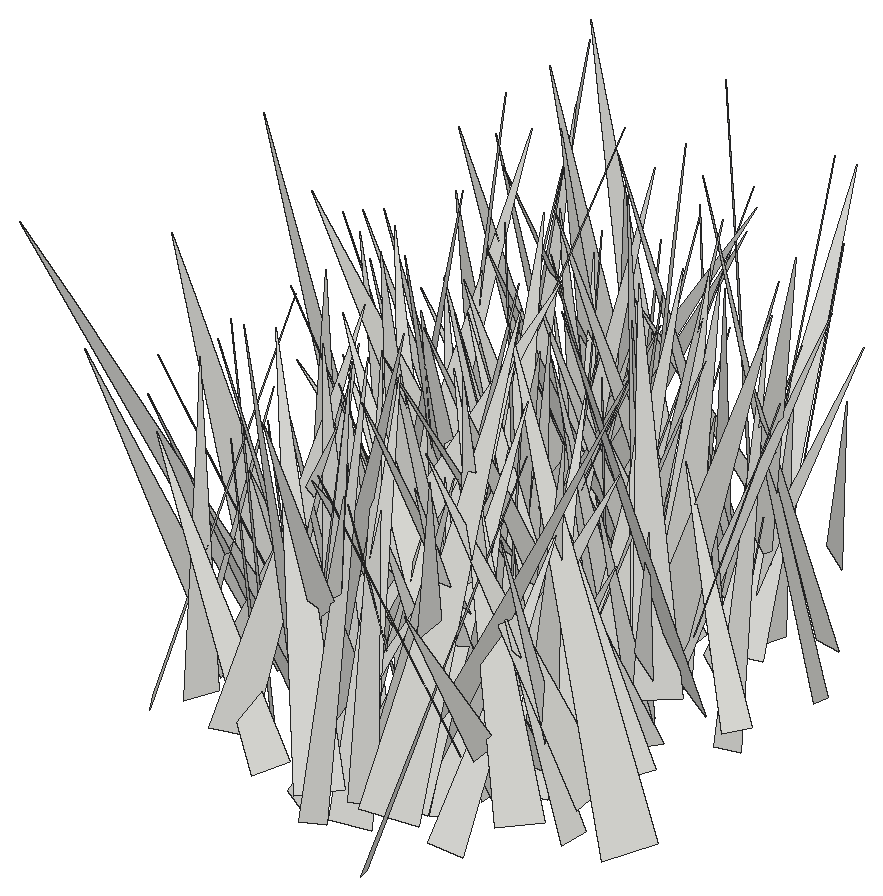
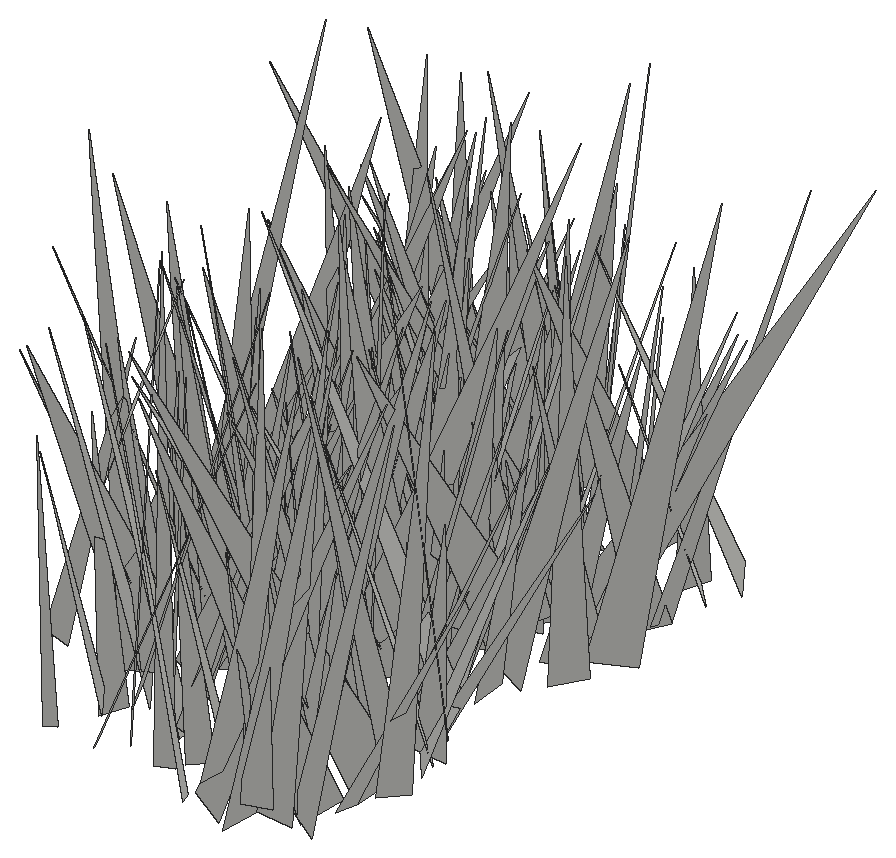
# SketchUp Ruby script. Lengths in inches.
U = 1.inch
M = Sketchup.active_model
def pt(a) = Geom::Point3d.new(a.map { |v| v * U })
def face(e, loops, mat)
  f = e.add_face(loops[0].map { |a| pt(a) })
  loops[1..].each { |l| e.add_face(l.map { |a| pt(a) }).erase! }
  f.material = f.back_material = mat if mat
  f
end
# faces: each face lists its corners as indices into pts; further lists are holes
def faces(e, pts, list, mat = nil) = list.each { |f| face(e, (f[0].is_a?(Array) ? f : [f]).map { |l| l.map { |i| pts[i] } }, mat) }
# xy, xz, yz: faces in a plane at the given z, y or x. An outline is a flat list of corners, or four numbers for a rectangle; further outlines are holes
def ring(l) = l.size == 4 ? [[l[0], l[1]], [l[2], l[1]], [l[2], l[3]], [l[0], l[3]]] : l.each_slice(2).to_a
def flat(e, list, mat, &to3) = list.each { |f| face(e, (f[0].is_a?(Array) ? f : [f]).map { |l| ring(l).map { |u, v| to3.(u, v) } }, mat) }
def xy(e, z, list, mat = nil) = flat(e, list, mat) { |x, y| [x, y, z] }
def xz(e, y, list, mat = nil) = flat(e, list, mat) { |x, z| [x, y, z] }
def yz(e, x, list, mat = nil) = flat(e, list, mat) { |y, z| [x, y, z] }
def lines(e, pts, list) = list.each { |a, b| e.add_line(pt(pts[a]), pt(pts[b])) }
# prism: a flat outline (further loops are holes) pulled along v
def prism(e, loops, v, mat = nil)
  f = face(e, loops, mat); d = Geom::Vector3d.new(v.map { |x| x * U })
  f.pushpull(f.normal.samedirection?(d) ? d.length : -d.length)
end
def box(e, o, s, mat = nil) = prism(e, [[o, [o[0] + s[0], o[1], o[2]], [o[0] + s[0], o[1] + s[1], o[2]], [o[0], o[1] + s[1], o[2]]]], [0, 0, s[2]], mat)
def at(x, y, z, deg = 0) = Geom::Transformation.translation(pt([x, y, z])) * Geom::Transformation.rotation(ORIGIN, Z_AXIS, deg.degrees)
def axes(o, x, y, z) = Geom::Transformation.new([*x, 0, *y, 0, *z, 0, *pt(o).to_a, 1])
def part(name) = M.definitions.add(name)
# library, detail: a bought-in or finely detailed component or shape, given as its bounding box
def library(name, o, s) = part(name).tap { |d| box(d.entities, o, s) }
def detail(e, o, s) = box(e.add_group.entities, o, s)
def put(e, d, t, mat = nil) = e.add_instance(d, t).tap { |i| i.material = mat if mat }
def group(e, t, mat = nil) = e.add_group.tap { |g| g.transformation = t; g.material = mat if mat }.entities
root = M.entities
c1 = part("fur_instance\#9")
p = [[0.8125,0,1.79],[0.67,-0.02,1.48],[0,-0.11,0],[0,0.11,0]]
faces(c1.entities,p,[[0,1,2,3]])
put(root,c1,axes([67.05,77.16,-27.1],[-1.39061,-8.04384,0.83594],[-7.45661,0.94696,-3.29214],[-3.13068,1.31752,7.46987]))
put(root,c1,axes([64.83,79.17,-27.1],[4.91943,-4.73173,2.30235],[-4.40019,-5.42749,-1.75256],[-2.8859,0.2095,6.59686]))
put(root,c1,axes([66.79,85.26,-28.22],[-4.61833,-3.74237,0.73758],[-3.79853,4.40694,-1.4242],[-0.34716,1.56584,5.77113]))
put(root,c1,axes([65.1875,76.49,-27.1],[-6.16239,-2.08969,1.53365],[-1.42213,6.03269,2.50561],[2.16712,-1.98337,6.00531]))
put(root,c1,axes([66.03,78.65,-27.1],[-3.26059,-4.43586,0.10579],[-4.43536,3.26207,0.0775],[0.12511,0.03932,5.50476]))
put(root,c1,axes([66.9375,81.38,-27.1],[-2.69995,-7.06667,2.40673],[-7.39529,2.18224,-1.88876],[-1.01973,2.88442,7.32531]))
put(root,c1,axes([66.75,88.64,-28.22],[-4.32306,0.06447,0.02072],[0.06687,4.27292,0.65655],[0.01068,-0.65679,4.2734]))
put(root,c1,axes([66.48,82.625,-27.1],[-5.31115,0.249,1.00047],[0.14264,5.37711,-0.58108],[1.02108,0.54405,5.28514]))
put(root,c1,axes([67.13,84.4,-28.22],[-4.70731,-0.314,0.0439],[-0.28456,4.4722,1.47573],[0.13983,-1.46975,4.48103]))
put(root,c1,axes([67.86,85.51,-28.22],[-6.00367,-1.40851,0.07652],[-1.40991,5.98159,-0.51624],[-0.04369,0.52005,6.14503]))
put(root,c1,axes([67.36,77.11,-28.22],[-2.53227,-4.93937,0.36335],[-4.86121,2.40071,-1.24381],[-0.94765,0.88376,5.4095]))
put(root,c1,axes([65.32,74.46,-27.1],[3.04107,3.48011,0.59696],[3.3547,-3.09349,0.94446],[-1.10161,0.1866,4.52408]))
put(root,c1,axes([65.85,74.29,-27.1],[-4.75498,1.70819,1.94206],[1.76287,5.11453,-0.18234],[1.89256,-0.47231,5.04921]))
put(root,c1,axes([66.79,84.88,-28.22],[-0.91318,4.58049,0.90258],[4.61205,0.74242,0.89849],[-0.72428,-1.04754,4.5834]))
put(root,c1,axes([65,73.07,-27.1],[5.18703,3.91751,0.7095],[3.72248,-5.18551,1.41748],[-1.41191,0.72053,6.34373]))
put(root,c1,axes([64.89,88.83,-27.1],[6.40589,-1.32849,1.4611],[-0.83624,-6.31798,-2.07823],[-1.78897,-1.80373,6.20333]))
put(root,c1,axes([65.13,80.71,-27.1],[5.79339,-2.08626,1.56673],[-1.97661,-6.00002,-0.68061],[-1.70297,-0.13319,6.11985]))
put(root,c1,axes([67.12,90.14,-28.22],[-3.32824,-5.52708,1.61735],[-5.74671,3.30884,-0.51825],[0.37393,1.65668,6.43096]))
put(root,c1,axes([67.9,75.06,-28.22],[-4.69579,-3.74143,2.09942],[-4.25802,4.44495,-1.60248],[0.52452,2.58851,5.78625]))
put(root,c1,axes([66.11,78.47,-27.1],[0.58745,4.61701,1.14714],[4.75417,-0.52722,-0.31264],[0.17496,-1.17604,4.64372]))
put(root,c1,axes([66.54,86.9,-27.1],[6.51752,3.06728,2.32468],[2.5593,-6.86862,1.88745],[-2.87443,0.8392,6.95153]))
put(root,c1,axes([68.79,73.77,-28.22],[-4.48303,2.72425,0.35571],[2.72908,4.33728,1.17718],[-0.3165,-1.18832,5.11208]))
put(root,c1,axes([66.82,75.65,-27.1],[-2.76326,-3.0585,1.38467],[-3.15346,2.97986,0.28892],[1.15213,0.82059,4.11176]))
put(root,c1,axes([68.75,81.83,-28.22],[-3.88022,2.75048,0.41463],[2.75578,3.70465,1.21426],[-0.37781,-1.22622,4.59857]))
put(root,c1,axes([67.08,84.48,-28.22],[4.3588,4.87451,1.02077],[4.50794,-4.43827,1.9448],[-2.11691,0.58556,6.24322]))
put(root,c1,axes([68.4375,84.53,-28.22],[-6.28754,-2.52373,1.27093],[-2.51372,6.41179,0.29625],[1.29062,0.19325,6.76865]))
put(root,c1,axes([66.24,84.8125,-27.1],[5.70767,4.90783,2.44546],[5.23724,-5.92496,-0.33273],[-1.62433,-1.85811,7.52021]))
put(root,c1,axes([67.25,78.6,-28.22],[3.46395,-3.11936,0.86631],[-2.7787,-3.51575,-1.54862],[-1.66124,-0.62369,4.39672]))
put(root,c1,axes([68.02,78.52,-27.1],[-3.33951,2.40161,0.05247],[2.31618,3.24301,-1.02031],[0.63702,0.79874,3.98485]))
put(root,c1,axes([67.73,85.81,-28.22],[1.84085,7.01016,1.12106],[6.97031,-2.00445,1.08846],[-1.34679,-0.79226,7.16563]))
put(root,c1,axes([67.9,82.61,-28.22],[-4.76858,-5.56642,0.65425],[-5.40433,4.79429,1.40014],[1.48534,-0.42682,7.19472]))
put(root,c1,axes([65.24,76.84,-27.1],[2.87453,-4.20489,0.68169],[-4.14129,-2.56592,1.63539],[0.99777,1.46412,4.82385]))
put(root,c1,axes([68.03,79.56,-27.1],[-6.65412,4.03174,0.74119],[3.28122,6.08544,-3.64454],[2.45722,2.79179,6.87384]))
put(root,c1,axes([68.76,87.92,-27.1],[-0.74223,-7.02206,1.66779],[-7.14663,0.48084,-1.156],[-1.00829,1.76103,6.96591]))
put(root,c1,axes([68.6,91.08,-28.22],[6.73753,-0.02978,4.19134],[0.53715,-7.86314,-0.91932],[-4.15689,-1.06433,6.67458]))
put(root,c1,axes([69.54,90.71,-27.1],[-7.31689,1.04904,1.18508],[0.99417,7.40794,-0.41938],[1.23147,0.25252,7.3798]))
put(root,c1,axes([69.73,75.91,-28.22],[-5.59539,-3.44886,0.89561],[-3.54081,5.56848,-0.67808],[0.39927,1.05,6.53783]))
put(root,c1,axes([68.99,87.99,-28.22],[0.68239,3.8164,1.4602],[3.78451,-1.14857,1.23331],[-1.54098,-1.13076,3.67553]))
put(root,c1,axes([69.8,91.05,-28.22],[-3.16334,-6.14078,0.476],[-6.132,3.08971,-0.89149],[-0.57823,0.82883,6.8499]))
put(root,c1,axes([68.99,77.39,-27.1],[-4.42725,-2.60663,1.07476],[-2.66002,4.52485,0.01676],[0.93485,0.53053,5.13759]))
put(root,c1,axes([67.67,79.5,-27.1],[3.15596,1.30372,1.61225],[1.82364,-3.14251,-1.02861],[-0.98659,-1.6383,3.25603]))
put(root,c1,axes([68.04,90.39,-28.22],[-0.95753,-7.17721,1.84222],[-7.39469,1.0444,0.22542],[0.47406,1.79439,7.23729]))
put(root,c1,axes([67.81,73.16,-27.1],[-5.19171,3.73852,1.55221],[3.028,5.26206,-2.54592],[2.68647,1.29382,5.8693]))
put(root,c1,axes([67.7,76.61,-27.1],[-3.39488,-3.98848,1.56761],[-3.7052,3.73666,1.48306],[2.15333,0.14147,5.02331]))
put(root,c1,axes([69.28,82.42,-28.22],[-2.05359,-3.75931,0.63579],[-3.81243,2.01617,-0.39286],[-0.04503,0.74602,4.26559]))
put(root,c1,axes([68.51,90.42,-27.1],[-3.5127,-1.06556,1.8883],[-1.54789,3.74984,-0.76344],[1.51826,1.35772,3.59049]))
put(root,c1,axes([70.71,78.52,-27.1],[-2.20757,6.36235,0.08993],[6.1827,2.12231,1.62203],[-1.50393,-0.61421,6.5362]))
put(root,c1,axes([69.17,87.8,-27.1],[-0.51846,-5.08764,2.15235],[-5.51728,0.36879,-0.45728],[-0.27624,2.18298,5.0935]))
put(root,c1,axes([69.26,77.63,-28.22],[1.73924,-4.25815,2.51532],[-4.74882,-2.1825,-0.41111],[-1.38108,2.14207,4.58125]))
put(root,c1,axes([69.03,76.91,-28.22],[-4.56803,3.68378,2.77525],[4.20348,4.93276,0.37129],[1.89817,-2.05836,5.85656]))
put(root,c1,axes([70.29,86.01,-28.22],[-4.8792,2.06982,0.10093],[1.96371,4.70056,-1.46614],[0.66196,1.31208,5.09325]))
put(root,c1,axes([71,82.37,-27.1],[-7.92224,1.63819,2.17065],[2.33717,7.51957,2.85498],[1.39032,-3.306,7.56932]))
put(root,c1,axes([66.44,84.1,-27.1],[7.55875,3.30018,0.58934],[3.3113,-7.57673,-0.04195],[-0.52327,-0.27436,8.24768]))
put(root,c1,axes([67.67,88.88,-28.22],[1.53162,3.70831,1.75315],[4.01532,-0.97314,-1.44953],[0.83802,-2.1148,3.74116]))
put(root,c1,axes([67.52,91.69,-27.1],[-1.15928,-6.64992,1.1524],[-6.36185,1.46707,2.06591],[2.25307,0.72087,6.42631]))
put(root,c1,axes([69.5625,88.5,-27.1],[-1.29873,-6.18935,0.13887],[-6.18983,1.30082,0.08883],[0.11547,0.11765,6.32352]))
put(root,c1,axes([68.91,87.21,-28.22],[-4.37143,-2.8181,2.86453],[-3.24687,4.97094,-0.06453],[2.3675,1.61389,5.20067]))
put(root,c1,axes([70.03,79.97,-27.1],[-3.79874,-3.55526,0.6962],[-3.51199,3.8615,0.55657],[0.88909,0.06302,5.17306]))
put(root,c1,axes([69.2,74.84,-27.1],[6.14406,2.36607,3.59044],[3.36505,-6.54408,-1.44586],[-2.67694,-2.79567,6.42319]))
put(root,c1,axes([69.2,81.94,-28.22],[2.92591,-1.89098,1.19539],[-1.88086,-3.14489,-0.37117],[-1.21125,0.31559,3.46396]))
put(root,c1,axes([68.77,78.125,-28.22],[7.33246,2.99097,2.42144],[2.72494,-7.71469,1.27771],[-2.71735,0.33456,7.81527]))
put(root,c1,axes([68.36,85.03,-28.22],[3.46775,1.51161,0.84573],[1.722,-3.21287,-1.3182],[-0.18693,-1.55498,3.54578]))
put(root,c1,axes([70.68,85.07,-27.1],[-5.0365,1.95588,2.0654],[2.56555,4.93734,1.5806],[1.22852,-2.29236,5.16658]))
put(root,c1,axes([69.53,80.25,-27.1],[4.70734,-3.12135,0.14145],[-2.64852,-4.12178,-2.81392],[-1.65776,-2.27815,4.89732]))
put(root,c1,axes([69.51,85.32,-28.22],[1.8777,6.7714,0.98346],[6.8334,-1.90815,0.09124],[-0.35155,-0.923,7.02632]))
put(root,c1,axes([71.98,71.98,-27.1],[-5.31881,4.24046,0.31909],[4.24772,5.322,0.07866],[0.20039,-0.26047,6.80184]))
put(root,c1,axes([69.96,79.34,-28.22],[2.83404,-7.21043,2.36501],[-7.48804,-3.06648,-0.37599],[-1.22999,2.05469,7.73827]))
put(root,c1,axes([68.78,75.66,-28.22],[6.76883,1.43904,1.95286],[1.74836,-6.90673,-0.9705],[-1.68159,-1.38844,6.85171]))
put(root,c1,axes([67.14,89.23,-28.22],[6.30652,-2.10429,0.15189],[-2.07978,-6.12031,1.56194],[0.35446,1.52876,6.46224]))
put(root,c1,axes([68.85,82.71,-27.1],[6.56004,-2.8558,0.90961],[-2.50702,-6.42798,-2.10074],[-1.6425,-1.59457,6.83935]))
put(root,c1,axes([66.69,87.15,-28.22],[6.90826,-2.9112,0.5406],[-2.88435,-6.30625,2.89882],[0.66922,2.87186,6.91346]))
put(root,c1,axes([70.875,79.46,-28.22],[1.62899,5.48386,2.82302],[6.01922,-2.05055,0.50999],[-1.34582,-2.53344,5.69792]))
put(root,c1,axes([69.9375,81.2,-27.1],[-3.5221,-6.63629,1.77015],[-6.5539,3.84233,1.36448],[2.0543,0.8804,7.38808]))
put(root,c1,axes([72.04,81.91,-27.1],[-1.46223,5.38545,2.28823],[5.73287,0.84616,1.67196],[-1.17188,-2.58033,5.32407]))
put(root,c1,axes([71.79,82.34,-27.1],[-4.56615,-2.82263,0.99228],[-2.92894,4.58662,-0.43101],[0.61084,0.89289,5.35081]))
put(root,c1,axes([70.79,81.26,-27.1],[-3.43213,5.64571,1.59286],[5.69776,3.64732,-0.65059],[1.39526,-1.00684,6.57497]))
put(root,c1,axes([68.89,84.77,-27.1],[4.92318,-0.35306,0.35659],[-0.43613,-4.74982,1.31852],[-0.24819,1.34315,4.75646]))
put(root,c1,axes([71.07,78.89,-28.22],[4.53649,3.63122,1.57008],[3.09166,-4.74451,2.04009],[-2.46831,0.73111,5.44092]))
put(root,c1,axes([70.17,76.09,-28.22],[2.21445,2.95218,0.72503],[3.03203,-2.20951,-0.26401],[-0.21871,-0.73996,3.68096]))
put(root,c1,axes([69.37,75.07,-28.22],[0.9975,-5.62203,0.93729],[-5.55991,-0.75041,1.41599],[1.25425,1.14473,5.53148]))
put(root,c1,axes([70.76,87.82,-27.1],[-3.28751,-5.48957,1.02333],[-5.33666,3.43821,1.29963],[1.64396,0.18343,6.2653]))
put(root,c1,axes([70.53,76.14,-28.22],[1.6119,-7.35068,0.1441],[-7.34568,-1.61634,-0.28263],[-0.30696,0.08011,7.52003]))
put(root,c1,axes([70.95,82.43,-28.22],[-4.9247,-5.05159,2.9073],[-5.39927,5.38751,0.21521],[2.19519,1.91829,7.05159]))
put(root,c1,axes([68.17,76.7,-27.1],[0.84349,7.5995,0.98427],[7.14395,-0.42161,-2.86687],[2.77222,-1.22577,7.08837]))
put(root,c1,axes([69.11,75.41,-27.1],[7.358,-0.55238,1.16955],[-0.51092,-7.44716,-0.30295],[-1.18825,-0.21839,7.37248]))
put(root,c1,axes([69.54,78.95,-28.22],[1.33461,3.80482,0.72121],[3.71713,-1.04467,-1.36733],[1.08616,-1.09999,3.79319]))
put(root,c1,axes([71.16,73.04,-27.1],[1.59622,5.71911,2.00108],[6.0184,-1.73595,0.16062],[-0.70101,-1.88115,5.93551]))
put(root,c1,axes([69.65,78.14,-28.22],[5.69643,3.12279,1.00252],[3.16084,-5.76326,-0.00802],[-0.87518,-0.48903,6.49623]))
put(root,c1,axes([72.21,86.69,-27.1],[-5.06877,-1.96642,0.89661],[-1.81084,5.11214,0.97466],[1.17965,-0.60192,5.34876]))
put(root,c1,axes([74.22,76.59,-28.22],[-5.71185,4.45959,0.23835],[4.39877,5.55102,1.55146],[-0.77178,-1.36683,7.07857]))
put(root,c1,axes([73.6,87.03,-27.1],[-0.2537,5.53184,2.90433],[5.7111,-0.97344,2.35297],[-2.53371,-2.74807,5.0129]))
put(root,c1,axes([72.73,78.67,-28.22],[-4.64621,2.31988,0.55706],[2.32982,4.67441,-0.03457],[0.51391,-0.21773,5.19306]))
put(root,c1,axes([71.46,85.68,-28.22],[3.22406,2.21993,1.84513],[2.48282,-3.54361,-0.0749],[-1.47248,-1.11442,3.91371]))
put(root,c1,axes([72.93,70.49,-27.1],[1.87355,6.48838,0.26131],[6.01197,-1.83596,2.48253],[-2.45429,0.45575,6.28063]))
put(root,c1,axes([70.1,84.7,-27.1],[4.41125,2.39111,1.26664],[2.67652,-4.21168,-1.37073],[-0.39751,-1.82353,4.82677]))
put(root,c1,axes([74.64,76.57,-28.22],[-7.75285,-2.01113,0.68817],[-2.11722,7.53738,-1.82488],[0.1887,1.94117,7.79879]))
put(root,c1,axes([72.93,88.29,-28.22],[-4.01235,0.08097,0.58825],[0.14386,4.03101,0.42638],[0.5761,-0.44265,3.99045]))
put(root,c1,axes([71.22,86.27,-28.22],[5.12051,1.66894,1.66295],[1.70709,-5.37015,0.13306],[-1.62376,-0.38277,5.38398]))
put(root,c1,axes([72.52,77.83,-28.22],[0.6809,-4.24063,0.83858],[-4.19337,-0.85411,-0.91428],[-1.04966,0.66131,4.19651]))
put(root,c1,axes([70.41,87.0625,-27.1],[4.87544,3.99495,1.42226],[4.19795,-4.85335,-0.75795],[-0.59966,-1.4959,6.2574]))
put(root,c1,axes([70.96,81.16,-28.22],[4.51704,3.2359,0.24642],[3.07452,-4.40221,1.45028],[-1.0388,1.04161,5.3639]))
put(root,c1,axes([73.36,72.23,-27.1],[1.09357,6.43106,0.77169],[6.11568,-1.28298,2.02542],[-2.13365,-0.38127,6.20097]))
put(root,c1,axes([72.75,84.74,-28.22],[-4.89796,-0.50596,1.28828],[-0.38248,5.0478,0.52832],[1.33018,-0.4116,4.8956]))
put(root,c1,axes([72.59,72.63,-28.22],[-0.70792,6.63222,0.94241],[6.69223,0.65809,0.39581],[-0.29764,-0.97786,6.65814]))
put(root,c1,axes([71.23,88.66,-27.1],[3.50621,1.98379,0.78234],[2.0421,-3.55715,-0.13217],[-0.61424,-0.50223,4.02634]))
put(root,c1,axes([70.33,77.07,-28.22],[4.54931,-2.96003,1.24819],[-3.21199,-4.22741,1.68171],[-0.05363,2.09362,5.16041]))
put(root,c1,axes([73.33,76.51,-27.1],[-3.18461,-4.17271,0.10236],[-4.17132,3.18622,0.10881],[0.1486,0.01532,5.24799]))
put(root,c1,axes([72.23,75.92,-27.1],[-3.11173,-3.4795,0.92655],[-3.33661,3.24675,0.98692],[1.3537,0.0043,4.56244]))
put(root,c1,axes([70.54,72.71,-28.22],[1.67584,3.97009,0.12724],[3.80521,-1.56498,-1.28741],[1.13936,-0.61275,4.1125]))
put(root,c1,axes([70.31,81.8,-28.22],[5.57249,-4.36069,0.56036],[-4.38496,-5.5781,0.19774],[-0.31889,0.50141,7.07313]))
put(root,c1,axes([74.07,88.83,-27.1],[-6.35383,-3.10693,1.06991],[-3.1587,6.41685,-0.12448],[0.9057,0.58302,7.07168]))
put(root,c1,axes([71.2,87.23,-28.22],[3.75751,0.05108,0.3502],[0.07903,-3.76142,-0.29936],[-0.34497,-0.30538,3.74592]))
put(root,c1,axes([75.03,84.4,-28.22],[-3.16767,-3.69393,0.44061],[-3.42422,2.66901,-2.24153],[-1.45395,1.76199,4.31912]))
put(root,c1,axes([73.25,91.72,-27.1],[-4.74866,-3.13825,0.27488],[-2.86364,4.50737,1.98925],[1.31291,-1.51952,5.33303]))
put(root,c1,axes([72.43,83.6,-27.1],[5.32818,4.49942,0.50618],[3.89144,-4.95023,3.04014],[-2.31467,2.03493,6.2763]))
put(root,c1,axes([73,90.46,-27.1],[-5.77727,-4.35757,2.82703],[-4.73437,6.15702,-0.18467],[2.13687,1.8601,7.23403]))
put(root,c1,axes([74.48,81.87,-27.1],[-4.28089,-1.18354,0.47624],[-1.27514,3.91753,-1.72642],[-0.03977,1.79046,4.09221]))
put(root,c1,axes([73.68,87.83,-28.22],[3.98122,4.30027,2.75674],[4.211,-4.74141,1.31475],[-2.89126,-0.98426,5.71085]))
put(root,c1,axes([75.57,81.36,-28.22],[-2.5504,-6.61055,0.06946],[-6.29815,2.40698,-2.17909],[-2.00934,0.84606,6.74207]))
put(root,c1,axes([73.69,86.86,-28.22],[-4.35378,0.44066,1.23045],[0.84047,4.2213,1.46212],[1.0009,-1.62788,4.12453]))
put(root,c1,axes([72.64,74.53,-28.22],[7.1916,2.06862,2.54607],[1.20326,-7.37063,2.58975],[-3.05186,1.96861,7.0208]))
put(root,c1,axes([72.9,74.61,-27.1],[-1.71935,6.00909,0.23442],[5.94835,1.73522,-0.85232],[0.8839,0.01135,6.19184]))
put(root,c1,axes([74.09,75.95,-27.1],[-3.60805,2.068,0.36238],[2.05277,3.62596,-0.25393],[0.44056,0.04128,4.15092]))
put(root,c1,axes([70.63,90.99,-28.22],[5.69332,3.04756,1.30745],[3.31373,-5.12843,-2.47574],[0.12746,-2.79687,5.96424]))
put(root,c1,axes([72.75,85.86,-27.1],[-2.53313,-4.37285,1.78451],[-4.47538,2.86942,0.67851],[1.50904,1.16947,5.00781]))
put(root,c1,axes([73.66,78.125,-27.1],[0.00503,4.167,0.7042],[4.17874,-0.11,0.62111],[-0.63075,-0.69557,4.12045]))
put(root,c1,axes([71.53,89.2,-28.22],[0.42063,-4.67833,0.35233],[-4.37367,-0.26302,1.72907],[1.69763,0.48155,4.36738]))
put(root,c1,axes([72.96,80.17,-27.1],[5.47635,-0.94494,2.24683],[-1.1073,-5.8869,0.22307],[-2.17142,0.61884,5.55279]))
put(root,c1,axes([74.93,83.07,-27.1],[-6.75602,-0.97126,1.58692],[-1.43223,6.52998,-2.10085],[1.1876,2.34979,6.49412]))
put(root,c1,axes([72.98,79.11,-27.1],[4.34542,2.75412,2.00138],[2.98226,-4.64462,-0.0836],[-1.6422,-1.14703,5.14401]))
put(root,c1,axes([77.11,77.49,-27.1],[-1.95645,6.57203,0.15793],[5.85701,1.66776,3.15567],[-2.98529,-1.03499,6.08778]))
put(root,c1,axes([74.61,79.26,-28.22],[-1.18349,4.29439,0.91251],[4.36217,1.04349,0.74676],[-0.49586,-1.06979,4.39144]))
put(root,c1,axes([75.09,75.77,-27.1],[-3.69691,-1.68274,0.52652],[-1.75981,3.59718,-0.85985],[0.10916,1.00233,3.96981]))
put(root,c1,axes([72.58,73.96,-27.1],[4.97792,-1.2009,1.19397],[-1.36113,-5.04298,0.6026],[-1.0075,0.87956,5.08515]))
put(root,c1,axes([74.54,74.71,-28.22],[-4.26385,3.34064,0.29483],[3.15748,4.15963,-1.468],[1.13011,0.98225,5.21395]))
put(root,c1,axes([74.64,82.53,-27.1],[5.18637,5.57386,2.23152],[5.04396,-5.64447,2.37581],[-3.2567,0.13438,7.23339]))
put(root,c1,axes([72.18,89.98,-28.22],[-2.5118,-6.70095,1.69222],[-6.07027,2.9998,2.86854],[3.30427,0.41708,6.55616]))
put(root,c1,axes([76.15,80.57,-28.22],[-0.7633,-7.78268,1.04828],[-7.63293,0.4877,-1.93706],[-1.84592,1.20152,7.57632]))
put(root,c1,axes([75.97,81.57,-28.22],[-4.45422,0.97791,0.2811],[1.01486,4.3608,0.91044],[0.07343,-0.95002,4.4685]))
put(root,c1,axes([75.9,76.9375,-27.1],[-1.54524,-6.7658,0.51217],[-6.71547,1.44992,-1.10738],[-0.96994,0.74015,6.85109]))
put(root,c1,axes([74.625,89.68,-27.1],[3.7445,3.22853,1.26331],[2.91821,-3.9391,1.41711],[-1.87174,0.31742,4.73672]))
put(root,c1,axes([74.49,81.52,-27.1],[-4.85985,3.92503,1.53679],[3.59209,5.08366,-1.6245],[2.20555,0.36911,6.032]))
put(root,c1,axes([74.71,82.02,-28.22],[-1.62337,4.08317,1.17277],[4.21606,1.70273,-0.09236],[0.52201,-1.05424,4.39307]))
put(root,c1,axes([74.625,81.8,-28.22],[4.10406,6.33899,0.98584],[6.11766,-4.2195,1.66374],[-1.93105,0.10466,7.36601]))
put(root,c1,axes([72.89,80.53,-28.22],[2.09245,-2.98815,0.44058],[-2.87886,-1.81085,1.39087],[0.91397,1.13723,3.37237]))
put(root,c1,axes([74.42,84.37,-28.22],[-0.45657,6.34549,1.8425],[6.59681,0.54314,-0.23589],[0.37708,-1.81886,6.35752]))
put(root,c1,axes([75.41,77.09,-28.22],[-2.14385,5.53708,0.23418],[5.53457,2.15208,-0.21752],[0.2875,-0.13964,5.93364]))
put(root,c1,axes([73.43,75.19,-27.1],[5.23311,-3.59302,0.50013],[-3.53385,-5.24745,-0.7222],[-0.81967,-0.31597,6.30664]))
put(root,c1,axes([73.93,79.88,-28.22],[-0.22733,-5.68785,1.31588],[-5.73337,0.46581,1.02292],[1.10075,1.2515,5.59972]))
put(root,c1,axes([74.43,72.85,-27.1],[-1.14169,6.19263,0.48775],[6.13199,1.20279,-0.91762],[0.99261,-0.30768,6.22978]))
put(root,c1,axes([74.9,76.26,-27.1],[1.62052,-5.44249,0.65001],[-5.43307,-1.68456,-0.55967],[-0.72449,0.45919,5.65098]))
put(root,c1,axes([73.47,81.4375,-27.1],[4.56753,3.50086,0.36537],[3.49009,-4.58212,0.27435],[-0.45689,-0.00383,5.74831]))
put(root,c1,axes([74.58,76.35,-27.1],[2.81734,-6.20209,1.85033],[-6.41792,-2.93797,-0.07572],[-0.83667,1.65211,6.81158]))
put(root,c1,axes([75.36,86.59,-28.22],[5.66789,4.81372,1.80284],[4.22946,-5.89252,2.43659],[-2.92126,0.80836,7.02566]))
put(root,c1,axes([74.63,70.69,-28.22],[5.4592,3.52611,0.65952],[3.05756,-5.20187,2.50265],[-1.87611,1.78282,5.99776]))
put(root,c1,axes([74.43,72.09,-27.1],[-3.17908,7.18759,1.82609],[7.05927,3.54175,-1.65087],[2.27218,-0.9472,7.68392]))
put(root,c1,axes([72.85,77.11,-28.22],[0.71966,5.69009,1.64056],[5.43341,0.02279,-2.46251],[2.35511,-1.79132,5.17987]))
put(root,c1,axes([72.92,88.1,-28.22],[5.75664,2.23558,0.62086],[2.31995,-5.52205,-1.62697],[0.03364,-1.74108,5.95732]))
put(root,c1,axes([76.32,81.46,-28.22],[1.33499,-4.14938,1.03511],[-3.92508,-1.61935,-1.42916],[-1.69781,0.48101,4.1179]))
put(root,c1,axes([76.11,82.17,-27.1],[-4.07853,4.6775,2.02917],[4.97181,4.22458,0.25488],[1.13033,-1.70436,6.20068]))
put(root,c1,axes([75.59,82.2,-28.22],[-3.9744,-0.24759,1.6573],[0.13335,4.20562,0.94807],[1.67038,-0.92483,3.8676]))
put(root,c1,axes([77.59,74.07,-27.1],[-3.01404,5.97197,0.86388],[5.95256,2.78442,1.51964],[-0.98886,-1.44144,6.51457]))
put(root,c1,axes([74.43,84.6,-28.22],[2.84119,-6.18581,2.36185],[-6.62137,-2.65127,1.02137],[0.00779,2.57322,6.73004]))
put(root,c1,axes([76.05,75.77,-27.1],[-1.30466,-3.28465,1.2487],[-3.51229,1.2605,-0.354],[0.10971,1.29326,3.5165]))
put(root,c1,axes([76.26,85.57,-27.1],[-5.16112,5.15909,0.10388],[4.87926,4.92701,-2.27629],[1.67923,1.54029,6.93338]))
put(root,c1,axes([75.29,88.37,-28.22],[4.19942,-1.36084,1.21546],[-1.38514,-4.36301,-0.09922],[-1.1877,0.2767,4.41329]))
put(root,c1,axes([75.97,76.2,-28.22],[4.06405,-3.6671,0.18626],[-3.28339,-3.75381,-2.26428],[-1.64366,-1.56845,4.98369]))
put(root,c1,axes([75.6,73.18,-28.22],[-1.59492,4.69203,0.53683],[4.53057,1.68008,-1.22409],[1.33316,-0.09626,4.80214]))
put(root,c1,axes([75.17,77.92,-28.22],[0.07384,-6.03784,2.03973],[-6.28438,0.27016,1.02718],[1.05955,2.02311,5.95028]))
put(root,c1,axes([75.18,82.58,-28.22],[0.57309,-4.07864,0.58369],[-4.03575,-0.43699,0.90892],[0.82985,0.69149,4.01716]))
put(root,c1,axes([74.89,91.71,-27.1],[-1.05562,-3.90874,0.84941],[-3.49411,1.32871,1.77194],[1.94702,0.26528,3.64044]))
put(root,c1,axes([78.18,76.66,-27.1],[-6.07615,0.58264,0.90457],[0.83184,5.83413,1.82981],[0.68247,-1.92372,5.8233]))
put(root,c1,axes([79.77,85.01,-27.1],[-7.1733,-2.93015,0.73361],[-2.97558,6.52972,-3.01478],[-0.51951,3.05896,7.13815]))
put(root,c1,axes([76.93,84.23,-28.22],[1.82668,3.73793,1.95155],[3.99067,-2.21946,0.51574],[-1.36206,-1.48974,4.1283]))
put(root,c1,axes([73.91,73.6,-27.1],[7.28902,-0.71217,0.57332],[-0.83779,-7.04721,1.89755],[-0.36604,1.94818,7.07364]))
put(root,c1,axes([74.9,86.12,-28.22],[3.15484,4.86518,0.39731],[4.85003,-3.07066,-0.91053],[0.55227,-0.82578,5.72659]))
put(root,c1,axes([78.45,78.61,-27.1],[-1.80359,3.13263,0.44398],[3.00697,1.53819,1.36218],[-0.98418,-1.04117,3.34825]))
put(root,c1,axes([76.8,82.87,-27.1],[-3.41876,-7.6362,0.72671],[-7.48826,3.49493,1.49637],[1.66304,0.03883,8.23167]))
put(root,c1,axes([74.87,83.64,-27.1],[5.22316,-4.20753,1.34718],[-4.41725,-5.01042,1.47756],[-0.07792,1.998,6.54228]))
put(root,c1,axes([77.36,76.45,-27.1],[-4.25466,-1.2014,1.34721],[-0.93808,4.41863,0.97784],[1.54219,-0.62673,4.31153]))
put(root,c1,axes([79.78,76.33,-28.22],[-7.19785,3.45896,0.52945],[3.49375,7.17168,0.64382],[0.19618,-0.81015,7.95983]))
put(root,c1,axes([74.83,87.66,-27.1],[0.15208,-7.64456,1.76209],[-7.47072,0.39677,2.36609],[2.3943,1.72356,7.27077]))
put(root,c1,axes([75.23,84.06,-27.1],[3.93505,4.96293,0.50565],[4.97977,-3.8695,-0.7745],[0.29702,-0.87596,6.28613]))
put(root,c1,axes([78.04,75.98,-28.22],[-3.68845,0.83243,0.84341],[0.99836,3.66829,0.74556],[0.6384,-0.92717,3.70698]))
put(root,c1,axes([78.22,82.71,-28.22],[1.43264,6.02249,0.66756],[5.77311,-1.565,1.72927],[-1.84042,-0.22107,5.94411]))
put(root,c1,axes([77.93,87.63,-27.1],[-1.24841,-4.57565,0.91997],[-4.66472,1.19209,-0.401],[-0.15278,0.99186,4.72592]))
put(root,c1,axes([78.98,82.1875,-27.1],[-2.26305,3.25436,0.20739],[3.19812,2.16563,0.91504],[-0.63708,-0.68879,3.8568]))
